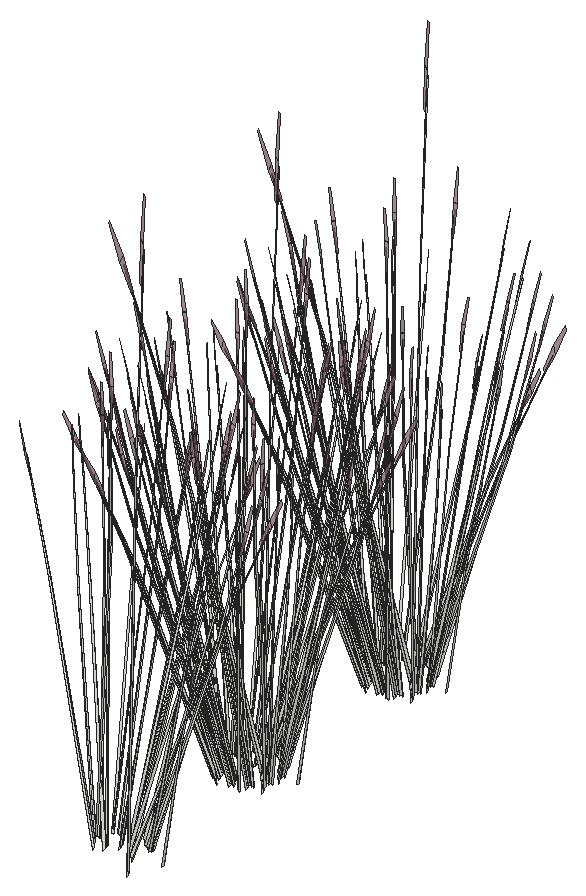
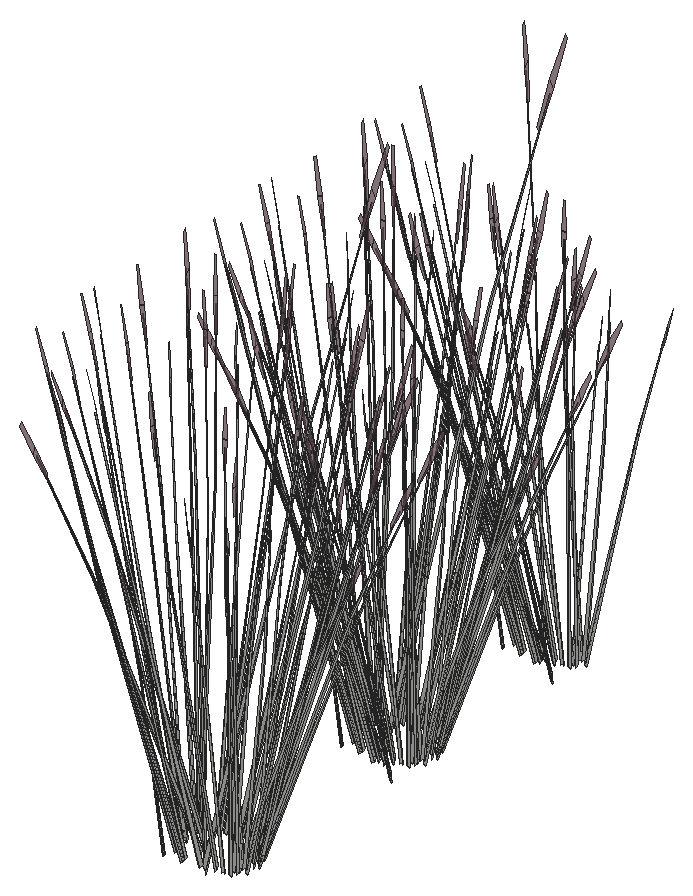
# SketchUp Ruby script. Lengths in inches.
U = 1.inch
M = Sketchup.active_model
def pt(a) = Geom::Point3d.new(a.map { |v| v * U })
def face(e, loops, mat)
  f = e.add_face(loops[0].map { |a| pt(a) })
  loops[1..].each { |l| e.add_face(l.map { |a| pt(a) }).erase! }
  f.material = f.back_material = mat if mat
  f
end
# faces: each face lists its corners as indices into pts; further lists are holes
def faces(e, pts, list, mat = nil) = list.each { |f| face(e, (f[0].is_a?(Array) ? f : [f]).map { |l| l.map { |i| pts[i] } }, mat) }
# xy, xz, yz: faces in a plane at the given z, y or x. An outline is a flat list of corners, or four numbers for a rectangle; further outlines are holes
def ring(l) = l.size == 4 ? [[l[0], l[1]], [l[2], l[1]], [l[2], l[3]], [l[0], l[3]]] : l.each_slice(2).to_a
def flat(e, list, mat, &to3) = list.each { |f| face(e, (f[0].is_a?(Array) ? f : [f]).map { |l| ring(l).map { |u, v| to3.(u, v) } }, mat) }
def xy(e, z, list, mat = nil) = flat(e, list, mat) { |x, y| [x, y, z] }
def xz(e, y, list, mat = nil) = flat(e, list, mat) { |x, z| [x, y, z] }
def yz(e, x, list, mat = nil) = flat(e, list, mat) { |y, z| [x, y, z] }
def lines(e, pts, list) = list.each { |a, b| e.add_line(pt(pts[a]), pt(pts[b])) }
# prism: a flat outline (further loops are holes) pulled along v
def prism(e, loops, v, mat = nil)
  f = face(e, loops, mat); d = Geom::Vector3d.new(v.map { |x| x * U })
  f.pushpull(f.normal.samedirection?(d) ? d.length : -d.length)
end
def box(e, o, s, mat = nil) = prism(e, [[o, [o[0] + s[0], o[1], o[2]], [o[0] + s[0], o[1] + s[1], o[2]], [o[0], o[1] + s[1], o[2]]]], [0, 0, s[2]], mat)
def at(x, y, z, deg = 0) = Geom::Transformation.translation(pt([x, y, z])) * Geom::Transformation.rotation(ORIGIN, Z_AXIS, deg.degrees)
def axes(o, x, y, z) = Geom::Transformation.new([*x, 0, *y, 0, *z, 0, *pt(o).to_a, 1])
def part(name) = M.definitions.add(name)
# library, detail: a bought-in or finely detailed component or shape, given as its bounding box
def library(name, o, s) = part(name).tap { |d| box(d.entities, o, s) }
def detail(e, o, s) = box(e.add_group.entities, o, s)
def put(e, d, t, mat = nil) = e.add_instance(d, t).tap { |i| i.material = mat if mat }
def group(e, t, mat = nil) = e.add_group.tap { |g| g.transformation = t; g.material = mat if mat }.entities
root = M.entities
M.materials.add("LightPink_Translucent").color = [144, 107, 117]
M.materials["LightPink_Translucent"].alpha = 0.75
c1 = part("blade")
p = [[2.15,0.21,22],[0,0.17,0],[0.09,0.45,0],[2.18,0.31,22],[2.29,0.31,22],[0.38,0.45,0],
  [2.48,0.24,33],[2.49,0.24,33],[2.48,0.22,33]]
faces(c1.entities,p,[[0,1,2,3],[4,5,2,3],[6,3,4,7],[8,0,3,6]])
c2 = part("seeds")
p = [[0.3,-0.1,1.38],[-0.01,-0.03,1.59],[-0.01,-0.03,0.03],[0.14,-0.07,-0.07],[0.29,-0.03,3],[0.15,0.01,3.11]]
faces(c2.entities,p,[[0,1,2,3],[1,0,4,5]],"LightPink_Translucent")
c3 = part("blade with seeds")
put(c3.entities,c1,at(0,0,0))
put(c3.entities,c2,axes([2.4,0.25,30.99],[1.5799,-0.05474,1.17369],[-0.12525,1.92788,0.29478],[-0.07173,-0.02425,1.56792]))
put(root,c3,axes([338.5,79.27,267.66],[-0.09788,-0.45691,-0.03251],[0.46264,-0.10504,-0.14742],[0.09661,0.02897,0.48626]))
put(root,c3,axes([337.3,79.26,268.6875],[0.02738,-0.55277,-0.11324],[0.51847,0.01511,-0.62851],[0.19968,0.0384,0.95501]))
put(root,c3,axes([333.43,77.8125,267.61],[0.17745,-0.11497,1.59586],[0.14939,0.53127,0.12904],[-0.27857,0.12007,0.68222]))
put(root,c3,axes([337.33,78.99,268.64],[0.51122,0.01309,-0.66157],[-0.03434,0.5511,0.07984],[0.21658,0.05816,0.93586]))
put(root,c3,axes([337.63,79.22,268.22],[0.29098,0.34031,-0.32977],[-0.33226,0.32215,0.42575],[0.16881,0.04902,0.81462]))
put(root,c3,axes([333.31,78.61,268.22],[-0.44516,0.07768,-0.32977],[-0.11755,-0.44407,0.42575],[-0.12757,0.11927,0.81462]))
put(root,c3,axes([336.59,78.35,267.61],[-0.18996,-0.09365,1.59586],[0.39312,-0.39287,0.12904],[0.24502,0.17723,0.68222]))
put(root,c3,axes([333.44,78.3,268.6875],[0.47307,0.29971,-0.11324],[-0.27254,0.43404,-0.62851],[-0.13365,0.15087,0.95501]))
put(root,c3,axes([336.28,79.86,268.6875],[0.30474,-0.46525,-0.11324],[0.44133,0.26804,-0.62851],[0.15341,0.13145,0.95501]))
put(root,c3,axes([334.08,78.17,267.61],[0.12773,-0.16701,1.59586],[0.32252,0.4508,0.12904],[-0.22121,0.20529,0.68222]))
put(root,c3,axes([333.67,78.66,268.36],[0.13138,0.49631,-0.47583],[-0.49754,0.08682,-0.36857],[-0.14258,0.13331,0.91046]))
put(root,c3,axes([336.59,77.65,266.65],[-0.01397,-0.51177,1.31553],[0.63227,0.13266,0.557],[-0.14954,0.28003,1.24175]))
put(root,c3,axes([336.64,79.63,268.36],[0.50465,-0.12921,-0.47583],[0.08828,0.48932,-0.36857],[0.13555,0.14022,0.91046]))
put(root,c3,axes([333.98,78.58,267.61],[0.09522,-0.18683,1.59586],[0.39947,0.38663,0.12904],[-0.18021,0.24097,0.68222]))
put(root,c3,axes([334.09,79.64,268.22],[-0.34603,0.28618,-0.32977],[-0.32756,-0.32677,0.42575],[-0.04984,0.16603,0.81462]))
put(root,c3,axes([335.09,79.875,268.6875],[0.50045,-0.25306,-0.11324],[0.24593,0.44915,-0.62851],[0.06603,0.18927,0.95501]))
put(root,c3,axes([334.44,79.5,268.66],[0.3661,0.36521,-0.52818],[-0.38674,0.31985,-0.40911],[-0.0557,0.18556,1.01061]))
put(root,c3,axes([335.52,79.85,268.36],[0.50273,0.13626,-0.47583],[-0.17232,0.46717,-0.36857],[0.0461,0.18809,0.91046]))
put(root,c3,axes([335.81,78.89,267.61],[-0.1169,-0.17452,1.59586],[0.54019,-0.14692,0.12904],[0.12209,0.27397,0.68222]))
put(root,c3,axes([335.29,80.14,268.22],[-0.15418,0.41799,-0.32977],[-0.44981,-0.12192,0.42575],[0.04124,0.16829,0.81462]))
put(root,c3,axes([334.32,79.33,268.97],[-0.01331,0.50278,-0.73435],[-0.56035,-0.03377,0.08862],[-0.05914,0.213,1.03881]))
put(root,c3,axes([334.85,78.98,267.61],[-0.01252,-0.20862,1.59586],[0.54251,0.1384,0.12904],[-0.03356,0.2973,0.68222]))
put(root,c3,axes([335.34,79.77,268.64],[0.24409,0.44196,-0.66157],[-0.50245,0.2463,0.07984],[0.05708,0.21354,0.93586]))
put(root,c3,axes([334.13,80.04,267.13],[0.01124,-0.2806,1.43727],[0.50537,0.14821,0.19862],[-0.04379,0.29905,0.67868]))
put(root,c3,axes([334.52,90.36,267.61],[0.1169,0.17452,1.59586],[-0.54019,0.14692,0.12904],[-0.12209,-0.27397,0.68222]))
put(root,c3,axes([335.96,90.49,268.64],[-0.24409,-0.44196,-0.66157],[0.50245,-0.2463,0.07984],[-0.05708,-0.21354,0.93586]))
put(root,c3,axes([336.98,90.92,268.64],[0.01331,-0.50278,-0.66157],[0.56035,0.03377,0.07984],[0.05914,-0.213,0.93586]))
put(root,c3,axes([336.01,90.11,268.22],[0.15418,-0.41799,-0.32977],[0.44981,0.12192,0.42575],[-0.04124,-0.16829,0.81462]))
put(root,c3,axes([336.35,90.67,267.61],[-0.09522,0.18683,1.59586],[-0.39947,-0.38663,0.12904],[0.18021,-0.24097,0.68222]))
put(root,c3,axes([335.78,90.4,268.36],[-0.50273,-0.13626,-0.47583],[0.17232,-0.46717,-0.36857],[-0.0461,-0.18809,0.91046]))
put(root,c3,axes([336.86,90.76,268.36],[-0.3661,-0.36521,-0.47583],[0.38674,-0.31985,-0.36857],[0.0557,-0.18556,0.91046]))
put(root,c3,axes([336.21,90.38,268.6875],[-0.50045,0.25306,-0.11324],[-0.24593,-0.44915,-0.62851],[-0.06603,-0.18927,0.95501]))
put(root,c3,axes([337.25,90.95,268.6875],[-0.56206,-0.02693,-0.11324],[0.01536,-0.50991,-0.62851],[0.03904,-0.19638,0.95501]))
put(root,c3,axes([337.21,90.62,268.22],[0.34603,-0.28618,-0.32977],[0.32756,0.32677,0.42575],[0.04984,-0.16603,0.81462]))
put(root,c3,axes([334.86,90.62,268.64],[-0.43608,-0.26272,-0.66157],[0.30991,-0.46038,0.07984],[-0.158,-0.15687,0.93586]))
put(root,c3,axes([334.71,90.27,268.22],[-0.07899,-0.43781,-0.32977],[0.45153,-0.11561,0.42575],[-0.12128,-0.12546,0.81462]))
put(root,c3,axes([333.74,90.9,267.61],[0.18996,0.09365,1.59586],[-0.39312,0.39287,0.12904],[-0.24502,-0.17723,0.68222]))
put(root,c3,axes([334.66,90.63,268.36],[-0.50465,0.12921,-0.47583],[-0.08828,-0.48932,-0.36857],[-0.13555,-0.14022,0.91046]))
put(root,c3,axes([337.64,91.8,268.64],[0.26714,-0.42887,-0.66157],[0.46811,0.30479,0.07984],[0.1595,-0.15539,0.93586]))
put(root,c3,axes([337.625,91.6,268.36],[-0.13138,-0.49631,-0.47583],[0.49754,-0.08682,-0.36857],[0.14258,-0.13331,0.91046]))
put(root,c3,axes([337.86,91.95,268.6875],[-0.47307,-0.29971,-0.11324],[0.27254,-0.43404,-0.62851],[0.13365,-0.15087,0.95501]))
put(root,c3,axes([335.91,93.59,267.1],[0.44194,0.21918,1.40854],[-0.43295,0.47219,0.557],[-0.19393,-0.27986,1.18082]))
put(root,c3,axes([337.99,91.65,268.22],[0.44516,-0.07768,-0.32977],[0.11755,0.44407,0.42575],[0.12757,-0.11927,0.81462]))
put(root,c3,axes([333.67,91.04,268.22],[-0.29098,-0.34031,-0.32977],[0.33226,-0.32215,0.42575],[-0.16881,-0.04902,0.81462]))
put(root,c3,axes([333.97,91.26,268.64],[-0.51122,-0.01309,-0.66157],[0.03434,-0.5511,0.07984],[-0.21658,-0.05816,0.93586]))
put(root,c3,axes([333.8,91.375,268.36],[-0.37135,0.36005,-0.47583],[-0.32522,-0.38035,-0.36857],[-0.18868,-0.05478,0.91046]))
put(root,c3,axes([334,91,268.6875],[-0.02738,0.55277,-0.11324],[-0.51847,-0.01511,-0.62851],[-0.19968,-0.0384,0.95501]))
put(root,c3,axes([337.88,93.12,268.6875],[-0.25732,-0.49218,-0.11324],[0.45669,-0.24187,-0.62851],[0.19245,-0.06494,0.95501]))
put(root,c3,axes([337.86,92.7,268.36],[0.13855,-0.49442,-0.47583],[0.47502,0.16947,-0.36857],[0.19125,-0.04534,0.91046]))
put(root,c3,axes([333.34,91.76,267.61],[0.21212,-0.01231,1.59586],[-0.14072,0.53355,0.12904],[-0.3023,-0.033,0.68222]))
put(root,c3,axes([337.77,92.88,268.64],[0.44939,-0.24006,-0.66157],[0.25044,0.49415,0.07984],[0.21713,-0.05613,0.93586]))
put(root,c3,axes([338.15,92.92,268.22],[0.42502,0.15163,-0.32977],[-0.12396,0.44238,0.42575],[0.17112,-0.04056,0.81462]))
put(root,c3,axes([333.15,92.22,268.22],[-0.42502,-0.15163,-0.32977],[0.12396,-0.44238,0.42575],[-0.17112,0.04056,0.81462]))
put(root,c3,axes([336.99,92.375,267.61],[-0.21212,0.01231,1.59586],[0.14072,-0.53355,0.12904],[0.3023,0.033,0.68222]))
put(root,c3,axes([334.45,92.15,267.11],[0.14537,-0.07863,1.64882],[0.05013,0.549,0.12904],[-0.31487,0.07285,0.5893]))
put(root,c3,axes([333.44,92.44,268.36],[-0.13855,0.49442,-0.47583],[-0.47502,-0.16947,-0.36857],[-0.19125,0.04534,0.91046]))
put(root,c3,axes([333.42,92.02,268.6875],[0.25732,0.49218,-0.11324],[-0.45669,0.24187,-0.62851],[-0.19245,0.06494,0.95501]))
put(root,c3,axes([338.5,94.16,267.66],[-0.09788,-0.45691,-0.03251],[0.46264,-0.10504,-0.14742],[0.09661,0.02897,0.48626]))
put(root,c3,axes([337.3,94.14,268.6875],[0.02738,-0.55277,-0.11324],[0.51847,0.01511,-0.62851],[0.19968,0.0384,0.95501]))
put(root,c3,axes([333.43,92.7,267.61],[0.17745,-0.11497,1.59586],[0.14939,0.53127,0.12904],[-0.27857,0.12007,0.68222]))
put(root,c3,axes([337.33,93.88,268.64],[0.51122,0.01309,-0.66157],[-0.03434,0.5511,0.07984],[0.21658,0.05816,0.93586]))
put(root,c3,axes([337.63,94.1,268.22],[0.29098,0.34031,-0.32977],[-0.33226,0.32215,0.42575],[0.16881,0.04902,0.81462]))
put(root,c3,axes([333.31,93.49,268.22],[-0.44516,0.07768,-0.32977],[-0.11755,-0.44407,0.42575],[-0.12757,0.11927,0.81462]))
put(root,c3,axes([336.59,93.23,267.61],[-0.18996,-0.09365,1.59586],[0.39312,-0.39287,0.12904],[0.24502,0.17723,0.68222]))
put(root,c3,axes([333.44,93.19,268.6875],[0.47307,0.29971,-0.11324],[-0.27254,0.43404,-0.62851],[-0.13365,0.15087,0.95501]))
put(root,c3,axes([336.28,94.74,268.6875],[0.30474,-0.46525,-0.11324],[0.44133,0.26804,-0.62851],[0.15341,0.13145,0.95501]))
put(root,c3,axes([334.08,93.06,267.61],[0.12773,-0.16701,1.59586],[0.32252,0.4508,0.12904],[-0.22121,0.20529,0.68222]))
put(root,c3,axes([333.67,93.55,268.36],[0.13138,0.49631,-0.47583],[-0.49754,0.08682,-0.36857],[-0.14258,0.13331,0.91046]))
put(root,c3,axes([336.59,92.54,266.65],[-0.01397,-0.51177,1.31553],[0.63227,0.13266,0.557],[-0.14954,0.28003,1.24175]))
put(root,c3,axes([336.64,94.51,268.36],[0.50465,-0.12921,-0.47583],[0.08828,0.48932,-0.36857],[0.13555,0.14022,0.91046]))
put(root,c3,axes([333.98,93.47,267.61],[0.09522,-0.18683,1.59586],[0.39947,0.38663,0.12904],[-0.18021,0.24097,0.68222]))
put(root,c3,axes([334.09,94.52,268.22],[-0.34603,0.28618,-0.32977],[-0.32756,-0.32677,0.42575],[-0.04984,0.16603,0.81462]))
put(root,c3,axes([335.09,94.76,268.6875],[0.50045,-0.25306,-0.11324],[0.24593,0.44915,-0.62851],[0.06603,0.18927,0.95501]))
put(root,c3,axes([334.44,94.39,268.66],[0.3661,0.36521,-0.52818],[-0.38674,0.31985,-0.40911],[-0.0557,0.18556,1.01061]))
put(root,c3,axes([335.52,94.74,268.36],[0.50273,0.13626,-0.47583],[-0.17232,0.46717,-0.36857],[0.0461,0.18809,0.91046]))
put(root,c3,axes([335.81,93.78,267.61],[-0.1169,-0.17452,1.59586],[0.54019,-0.14692,0.12904],[0.12209,0.27397,0.68222]))
put(root,c3,axes([335.29,95.03,268.22],[-0.15418,0.41799,-0.32977],[-0.44981,-0.12192,0.42575],[0.04124,0.16829,0.81462]))
put(root,c3,axes([334.32,94.22,268.97],[-0.01331,0.50278,-0.73435],[-0.56035,-0.03377,0.08862],[-0.05914,0.213,1.03881]))
put(root,c3,axes([334.85,93.86,267.61],[-0.01252,-0.20862,1.59586],[0.54251,0.1384,0.12904],[-0.03356,0.2973,0.68222]))
put(root,c3,axes([335.34,94.65,268.64],[0.24409,0.44196,-0.66157],[-0.50245,0.2463,0.07984],[0.05708,0.21354,0.93586]))
put(root,c3,axes([334.13,94.93,267.13],[0.01124,-0.2806,1.43727],[0.50537,0.14821,0.19862],[-0.04379,0.29905,0.67868]))
put(root,c3,axes([334.52,106.78,267.61],[0.1169,0.17452,1.59586],[-0.54019,0.14692,0.12904],[-0.12209,-0.27397,0.68222]))
put(root,c3,axes([335.96,106.91,268.64],[-0.24409,-0.44196,-0.66157],[0.50245,-0.2463,0.07984],[-0.05708,-0.21354,0.93586]))
put(root,c3,axes([336.98,107.34,268.64],[0.01331,-0.50278,-0.66157],[0.56035,0.03377,0.07984],[0.05914,-0.213,0.93586]))
put(root,c3,axes([336.01,106.53,268.22],[0.15418,-0.41799,-0.32977],[0.44981,0.12192,0.42575],[-0.04124,-0.16829,0.81462]))
put(root,c3,axes([336.35,107.09,267.61],[-0.09522,0.18683,1.59586],[-0.39947,-0.38663,0.12904],[0.18021,-0.24097,0.68222]))
put(root,c3,axes([335.78,106.82,268.36],[-0.50273,-0.13626,-0.47583],[0.17232,-0.46717,-0.36857],[-0.0461,-0.18809,0.91046]))
put(root,c3,axes([336.86,107.17,268.36],[-0.3661,-0.36521,-0.47583],[0.38674,-0.31985,-0.36857],[0.0557,-0.18556,0.91046]))
put(root,c3,axes([336.21,106.8,268.6875],[-0.50045,0.25306,-0.11324],[-0.24593,-0.44915,-0.62851],[-0.06603,-0.18927,0.95501]))
put(root,c3,axes([337.25,107.37,268.6875],[-0.56206,-0.02693,-0.11324],[0.01536,-0.50991,-0.62851],[0.03904,-0.19638,0.95501]))
put(root,c3,axes([337.21,107.04,268.22],[0.34603,-0.28618,-0.32977],[0.32756,0.32677,0.42575],[0.04984,-0.16603,0.81462]))
put(root,c3,axes([334.86,107.03,268.64],[-0.43608,-0.26272,-0.66157],[0.30991,-0.46038,0.07984],[-0.158,-0.15687,0.93586]))
put(root,c3,axes([334.71,106.6875,268.22],[-0.07899,-0.43781,-0.32977],[0.45153,-0.11561,0.42575],[-0.12128,-0.12546,0.81462]))
put(root,c3,axes([333.74,107.32,267.61],[0.18996,0.09365,1.59586],[-0.39312,0.39287,0.12904],[-0.24502,-0.17723,0.68222]))
put(root,c3,axes([334.66,107.05,268.36],[-0.50465,0.12921,-0.47583],[-0.08828,-0.48932,-0.36857],[-0.13555,-0.14022,0.91046]))
put(root,c3,axes([337.64,108.21,268.64],[0.26714,-0.42887,-0.66157],[0.46811,0.30479,0.07984],[0.1595,-0.15539,0.93586]))
put(root,c3,axes([337.625,108.01,268.36],[-0.13138,-0.49631,-0.47583],[0.49754,-0.08682,-0.36857],[0.14258,-0.13331,0.91046]))
put(root,c3,axes([337.86,108.37,268.6875],[-0.47307,-0.29971,-0.11324],[0.27254,-0.43404,-0.62851],[0.13365,-0.15087,0.95501]))
put(root,c3,axes([335.91,110.01,267.1],[0.44194,0.21918,1.40854],[-0.43295,0.47219,0.557],[-0.19393,-0.27986,1.18082]))
put(root,c3,axes([337.99,108.07,268.22],[0.44516,-0.07768,-0.32977],[0.11755,0.44407,0.42575],[0.12757,-0.11927,0.81462]))
put(root,c3,axes([333.67,107.46,268.22],[-0.29098,-0.34031,-0.32977],[0.33226,-0.32215,0.42575],[-0.16881,-0.04902,0.81462]))
put(root,c3,axes([333.97,107.68,268.64],[-0.51122,-0.01309,-0.66157],[0.03434,-0.5511,0.07984],[-0.21658,-0.05816,0.93586]))
put(root,c3,axes([333.8,107.79,268.36],[-0.37135,0.36005,-0.47583],[-0.32522,-0.38035,-0.36857],[-0.18868,-0.05478,0.91046]))
put(root,c3,axes([334,107.42,268.6875],[-0.02738,0.55277,-0.11324],[-0.51847,-0.01511,-0.62851],[-0.19968,-0.0384,0.95501]))
put(root,c3,axes([337.88,109.54,268.6875],[-0.25732,-0.49218,-0.11324],[0.45669,-0.24187,-0.62851],[0.19245,-0.06494,0.95501]))
put(root,c3,axes([337.86,109.12,268.36],[0.13855,-0.49442,-0.47583],[0.47502,0.16947,-0.36857],[0.19125,-0.04534,0.91046]))
put(root,c3,axes([333.34,108.18,267.61],[0.21212,-0.01231,1.59586],[-0.14072,0.53355,0.12904],[-0.3023,-0.033,0.68222]))
put(root,c3,axes([337.77,109.3,268.64],[0.44939,-0.24006,-0.66157],[0.25044,0.49415,0.07984],[0.21713,-0.05613,0.93586]))
put(root,c3,axes([338.15,109.34,268.22],[0.42502,0.15163,-0.32977],[-0.12396,0.44238,0.42575],[0.17112,-0.04056,0.81462]))
put(root,c3,axes([333.15,108.64,268.22],[-0.42502,-0.15163,-0.32977],[0.12396,-0.44238,0.42575],[-0.17112,0.04056,0.81462]))
put(root,c3,axes([336.99,108.79,267.61],[-0.21212,0.01231,1.59586],[0.14072,-0.53355,0.12904],[0.3023,0.033,0.68222]))
put(root,c3,axes([334.45,108.5625,267.11],[0.14537,-0.07863,1.64882],[0.05013,0.549,0.12904],[-0.31487,0.07285,0.5893]))
put(root,c3,axes([333.44,108.86,268.36],[-0.13855,0.49442,-0.47583],[-0.47502,-0.16947,-0.36857],[-0.19125,0.04534,0.91046]))
put(root,c3,axes([333.42,108.44,268.6875],[0.25732,0.49218,-0.11324],[-0.45669,0.24187,-0.62851],[-0.19245,0.06494,0.95501]))
put(root,c3,axes([338.5,110.58,267.66],[-0.09788,-0.45691,-0.03251],[0.46264,-0.10504,-0.14742],[0.09661,0.02897,0.48626]))
put(root,c3,axes([337.3,110.5625,268.6875],[0.02738,-0.55277,-0.11324],[0.51847,0.01511,-0.62851],[0.19968,0.0384,0.95501]))
put(root,c3,axes([333.43,109.12,267.61],[0.17745,-0.11497,1.59586],[0.14939,0.53127,0.12904],[-0.27857,0.12007,0.68222]))
put(root,c3,axes([337.33,110.3,268.64],[0.51122,0.01309,-0.66157],[-0.03434,0.5511,0.07984],[0.21658,0.05816,0.93586]))
put(root,c3,axes([337.63,110.52,268.22],[0.29098,0.34031,-0.32977],[-0.33226,0.32215,0.42575],[0.16881,0.04902,0.81462]))
put(root,c3,axes([333.31,109.91,268.22],[-0.44516,0.07768,-0.32977],[-0.11755,-0.44407,0.42575],[-0.12757,0.11927,0.81462]))
put(root,c3,axes([336.59,109.65,267.61],[-0.18996,-0.09365,1.59586],[0.39312,-0.39287,0.12904],[0.24502,0.17723,0.68222]))
put(root,c3,axes([333.44,109.61,268.6875],[0.47307,0.29971,-0.11324],[-0.27254,0.43404,-0.62851],[-0.13365,0.15087,0.95501]))
put(root,c3,axes([336.28,111.16,268.6875],[0.30474,-0.46525,-0.11324],[0.44133,0.26804,-0.62851],[0.15341,0.13145,0.95501]))
put(root,c3,axes([334.08,109.48,267.61],[0.12773,-0.16701,1.59586],[0.32252,0.4508,0.12904],[-0.22121,0.20529,0.68222]))
put(root,c3,axes([333.67,109.96,268.36],[0.13138,0.49631,-0.47583],[-0.49754,0.08682,-0.36857],[-0.14258,0.13331,0.91046]))
put(root,c3,axes([336.59,108.96,266.65],[-0.01397,-0.51177,1.31553],[0.63227,0.13266,0.557],[-0.14954,0.28003,1.24175]))
put(root,c3,axes([336.64,110.93,268.36],[0.50465,-0.12921,-0.47583],[0.08828,0.48932,-0.36857],[0.13555,0.14022,0.91046]))
put(root,c3,axes([333.98,109.89,267.61],[0.09522,-0.18683,1.59586],[0.39947,0.38663,0.12904],[-0.18021,0.24097,0.68222]))
put(root,c3,axes([334.09,110.94,268.22],[-0.34603,0.28618,-0.32977],[-0.32756,-0.32677,0.42575],[-0.04984,0.16603,0.81462]))
put(root,c3,axes([335.09,111.18,268.6875],[0.50045,-0.25306,-0.11324],[0.24593,0.44915,-0.62851],[0.06603,0.18927,0.95501]))
put(root,c3,axes([334.43,110.81,268.66],[0.3661,0.36521,-0.52818],[-0.38674,0.31985,-0.40911],[-0.0557,0.18556,1.01061]))
